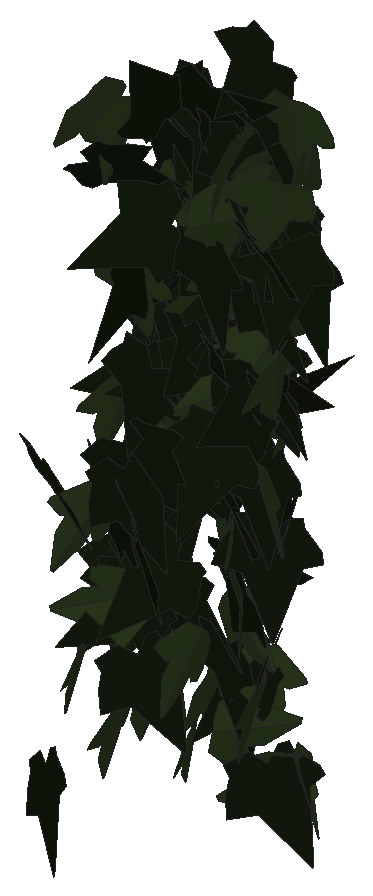
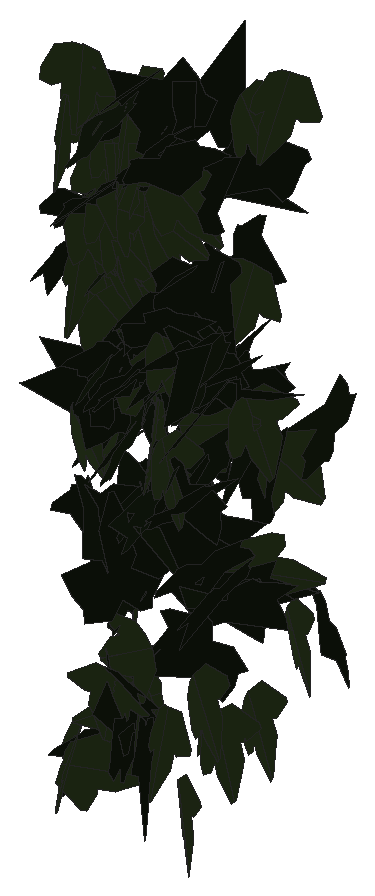
# SketchUp Ruby script. Lengths in inches.
U = 1.inch
M = Sketchup.active_model
def pt(a) = Geom::Point3d.new(a.map { |v| v * U })
def face(e, loops, mat)
  f = e.add_face(loops[0].map { |a| pt(a) })
  loops[1..].each { |l| e.add_face(l.map { |a| pt(a) }).erase! }
  f.material = f.back_material = mat if mat
  f
end
# faces: each face lists its corners as indices into pts; further lists are holes
def faces(e, pts, list, mat = nil) = list.each { |f| face(e, (f[0].is_a?(Array) ? f : [f]).map { |l| l.map { |i| pts[i] } }, mat) }
# xy, xz, yz: faces in a plane at the given z, y or x. An outline is a flat list of corners, or four numbers for a rectangle; further outlines are holes
def ring(l) = l.size == 4 ? [[l[0], l[1]], [l[2], l[1]], [l[2], l[3]], [l[0], l[3]]] : l.each_slice(2).to_a
def flat(e, list, mat, &to3) = list.each { |f| face(e, (f[0].is_a?(Array) ? f : [f]).map { |l| ring(l).map { |u, v| to3.(u, v) } }, mat) }
def xy(e, z, list, mat = nil) = flat(e, list, mat) { |x, y| [x, y, z] }
def xz(e, y, list, mat = nil) = flat(e, list, mat) { |x, z| [x, y, z] }
def yz(e, x, list, mat = nil) = flat(e, list, mat) { |y, z| [x, y, z] }
def lines(e, pts, list) = list.each { |a, b| e.add_line(pt(pts[a]), pt(pts[b])) }
# prism: a flat outline (further loops are holes) pulled along v
def prism(e, loops, v, mat = nil)
  f = face(e, loops, mat); d = Geom::Vector3d.new(v.map { |x| x * U })
  f.pushpull(f.normal.samedirection?(d) ? d.length : -d.length)
end
def box(e, o, s, mat = nil) = prism(e, [[o, [o[0] + s[0], o[1], o[2]], [o[0] + s[0], o[1] + s[1], o[2]], [o[0], o[1] + s[1], o[2]]]], [0, 0, s[2]], mat)
def at(x, y, z, deg = 0) = Geom::Transformation.translation(pt([x, y, z])) * Geom::Transformation.rotation(ORIGIN, Z_AXIS, deg.degrees)
def axes(o, x, y, z) = Geom::Transformation.new([*x, 0, *y, 0, *z, 0, *pt(o).to_a, 1])
def part(name) = M.definitions.add(name)
# library, detail: a bought-in or finely detailed component or shape, given as its bounding box
def library(name, o, s) = part(name).tap { |d| box(d.entities, o, s) }
def detail(e, o, s) = box(e.add_group.entities, o, s)
def put(e, d, t, mat = nil) = e.add_instance(d, t).tap { |i| i.material = mat if mat }
def group(e, t, mat = nil) = e.add_group.tap { |g| g.transformation = t; g.material = mat if mat }.entities
root = M.entities
M.materials.add("efeu1").color = [18, 25, 13]
M.materials.add("efeu2").color = [43, 57, 29]
c1 = part("ivyleaf_9")
p = [[1.54,2.16,1.25],[1.36,2.04,1.19],[-0.21,0.99,0.68],[-0.71,1.11,0.82],[-0.85,0.86,0.67],[-0.8,0.17,0.21],
  [-0.9,-0.01,0.1],[-0.67,-0.16,-0.02],[-0.08,-0.08,-0.05],[-0.03,-0.6,-0.4],[0.65,-0.88,-0.66],[0.83,-0.6,-0.49],
  [1.29,-0.42,-0.43],[1.8125,-0.07,-0.26],[1.21,0.44,0.15]]
faces(c1.entities,p,[[0,1,2,3,4,5,6,7,8,9,10,11,12,13,14]],"efeu1")
c2 = part("ivyleaf_10")
p = [[0,0.5,-0.03],[-0.0625,2.02,-0.43],[-0.19,2.01,-0.46],[-0.54,1.05,-0.29],[-0.52,0.625,-0.18],[-0.83,0.76,-0.28],
  [-1.16,0.64,-0.33],[-1.15,0.33,-0.24],[-0.77,-0.39,0.02],[-0.3,-0.51,0.16],[0.04,-0.48,0.23],[-0.02,2.01,-0.4375],
  [-0.06,2.01,-0.43],[0.04,-0.49,0.23],[0.67,-0.49,0.14],[1.38,0.36,-0.2],[1.375,0.51,-0.24],[0.81,0.65,-0.19],
  [0.62,0.59,-0.15],[0.6,1.09,-0.28],[0.5,1.23,-0.31]]
faces(c2.entities,p,[[0,1,2,3,4,5,6,7,8,9,10],[11,12,0,13,14,15,16,17,18,19,20]],"efeu2")
put(root,c1,axes([25.81,219.31,224.23],[-0.18904,-0.04184,-0.46099],[0.46288,-0.01554,-0.1884],[0.00144,-0.498,0.04461]))
put(root,c2,axes([27.44,220.39,226.23],[-0.01379,-0.37116,0.33473],[0.11301,-0.32851,-0.3596],[0.48687,0.06574,0.09295]))
put(root,c1,axes([26.5625,220.48,227.02],[0.04822,-0.11383,0.48448],[0.15449,-0.45927,-0.12329],[0.47308,0.16159,-0.00912]))
put(root,c1,axes([24.8,220.53,228.01],[0.28782,-0.34234,0.22352],[0.138,-0.17596,-0.44721],[0.38486,0.31912,-0.0068]))
put(root,c2,axes([25.41,220.82,227.49],[-0.09514,-0.36129,0.33229],[0.00188,-0.33874,-0.36777],[0.49086,-0.06873,0.06582]))
put(root,c1,axes([26.41,220.55,225.6],[0.03321,-0.38306,-0.31963],[0.02396,0.32119,-0.38244],[0.49832,0.01008,0.03969]))
put(root,c1,axes([26.13,220.63,228.31],[0.07521,-0.41705,-0.26536],[-0.03138,0.26384,-0.42356],[0.49331,0.08037,0.01351]))
put(root,c2,axes([25.125,220.91,225.13],[0.22225,-0.44783,-0.00737],[-0.00287,0.0068,-0.49995],[0.44788,0.22227,0.00045]))
put(root,c1,axes([26,220.79,228.62],[-0.06742,-0.1291,-0.47832],[0.19906,0.43499,-0.14546],[0.45369,-0.21004,-0.00726]))
put(root,c1,axes([25.79,220.86,228.05],[0.39057,-0.12931,-0.28413],[-0.27142,0.08416,-0.4114],[0.15422,0.4756,-0.00445]))
put(root,c2,axes([25.64,221.24,225.96],[0.10725,0.03356,-0.48721],[-0.44387,-0.20131,-0.11158],[-0.20365,0.45645,-0.01339]))
put(root,c1,axes([25.75,221,226.95],[0.16378,-0.2526,0.39921],[-0.16659,0.3645,0.29898],[-0.44207,-0.23094,0.03524]))
put(root,c1,axes([26.95,221.34,231.67],[0.14266,-0.47158,0.08521],[0.0193,-0.08318,-0.49265],[0.47883,0.14385,-0.00553]))
put(root,c1,axes([26.23,221.37,231.82],[-0.43879,-0.09642,0.21947],[-0.2121,-0.05714,-0.44916],[0.1117,-0.48728,0.00925]))
put(root,c1,axes([25.61,221.55,230.87],[-0.0735,0.05071,-0.49196],[0.3068,-0.38542,-0.08556],[-0.3879,-0.31445,0.02554]))
put(root,c2,axes([25.1,221.14,233.39],[-0.1399,-0.41319,-0.24434],[0.09004,0.2274,-0.4361],[0.47151,-0.16602,0.01078]))
put(root,c1,axes([25.71,221.68,229.26],[-0.04681,-0.44308,0.2269],[0.0125,-0.22888,-0.44436],[0.49765,-0.03592,0.0325]))
put(root,c1,axes([26.15,221.61,226.52],[-0.4073,-0.27121,0.10272],[-0.08761,-0.05376,-0.48932],[0.27646,-0.4166,-0.00373]))
put(root,c1,axes([25.68,221.7,225.74],[-0.29758,-0.24734,0.31665],[-0.23457,-0.21297,-0.38681],[0.32622,-0.37877,0.01071]))
put(root,c2,axes([25.38,221.55,233.18],[0.02209,-0.46526,0.18178],[0.06664,-0.17759,-0.46262],[0.49505,0.04466,0.05417]))
put(root,c2,axes([25.36,221.44,223.99],[0.1074,-0.48763,0.02618],[0.00063,-0.02667,-0.49929],[0.48833,0.10728,-0.00511]))
put(root,c1,axes([25.19,221.11,232.55],[0.40335,0.2125,0.2053],[0.17439,0.10923,-0.45569],[-0.23852,0.43922,0.014]))
put(root,c1,axes([26.89,221.72,228.6],[-0.34885,-0.35579,-0.04139],[0.02971,0.02884,-0.49828],[0.35696,-0.35012,0.00102]))
put(root,c1,axes([27.27,222.03,229.15],[-0.09536,-0.26151,0.41535],[-0.15206,-0.38656,-0.2783],[0.46667,-0.17939,-0.00581]))
put(root,c2,axes([26.94,221.83,232.96],[0.22417,-0.41973,0.15355],[0.07269,-0.13526,-0.47584],[0.44098,0.23566,0.00038]))
put(root,c2,axes([25.14,221.79,228.75],[-0.07663,-0.48144,0.1111],[-0.00512,-0.11164,-0.48735],[0.49407,-0.07582,0.01218]))
put(root,c2,axes([26.85,221.33,232.11],[-0.054,-0.09278,-0.48834],[0.24653,0.42155,-0.10735],[0.43163,-0.25237,0.00021]))
put(root,c2,axes([25.32,221.69,230.65],[-0.49774,0.00252,-0.04744],[0.04743,-0.00113,-0.49774],[-0.00261,-0.49999,0.00088]))
put(root,c1,axes([25.43,221.98,225.99],[-0.33292,-0.36474,-0.07828],[0.06171,0.04963,-0.49369],[0.36791,-0.33838,0.01197]))
put(root,c1,axes([25.68,222,233.05],[0.19902,0.17508,0.42395],[-0.30783,-0.29163,0.26494],[0.34005,-0.36647,-0.00829]))
put(root,c1,axes([25.25,222.11,225.99],[-0.31182,-0.37943,0.09381],[-0.05983,-0.07226,-0.49112],[0.38625,-0.3175,-0.00034]))
put(root,c2,axes([27.73,221.89,232.59],[-0.36147,-0.31379,0.14448],[-0.10382,-0.10077,-0.47861],[0.32949,-0.37601,0.00769]))
put(root,c2,axes([26,221.87,228.33],[-0.12966,0.03247,-0.4818],[-0.47823,0.06057,0.13278],[0.06699,0.49525,0.01535]))
put(root,c1,axes([25.49,221.99,228.27],[0.37885,-0.27455,0.17634],[0.14255,-0.1038,-0.46787],[0.29352,0.40478,-0.00037]))
put(root,c2,axes([27.35,222.04,227.98],[-0.29803,0.31399,-0.25018],[0.16913,-0.18439,-0.43289],[-0.36411,-0.34266,0.00369]))
put(root,c1,axes([26.65,222.28,229.24],[0.39155,-0.27756,-0.14019],[0.11367,-0.08207,0.47994],[-0.28943,-0.40771,-0.00117]))
put(root,c2,axes([26.75,222.13,231.03],[-0.07618,-0.48051,0.11535],[0.01731,-0.11923,-0.48527],[0.49386,-0.06994,0.0348]))
put(root,c1,axes([25.64,222.33,229.01],[-0.37326,-0.07606,0.32387],[-0.26354,-0.22947,-0.35762],[0.20304,-0.43767,0.13122]))
put(root,c2,axes([27.54,222.02,229.8],[0.04755,-0.47944,-0.13372],[0.0118,0.13538,-0.48118],[0.49759,0.0426,0.02419]))
put(root,c2,axes([27.16,222.29,232.44],[-0.04919,-0.44271,0.22713],[-0.0041,-0.22787,-0.44504],[0.49756,-0.04565,0.01879]))
put(root,c1,axes([27.33,222.35,231.21],[0.32566,-0.37936,0.00614],[0.00075,0.00873,0.49992],[-0.37941,-0.3256,0.00625]))
put(root,c2,axes([26.59,222.47,228.98],[-0.07324,0.02485,0.49398],[-0.05974,-0.49616,0.01611],[0.49099,-0.05666,0.07564]))
put(root,c1,axes([27.09,222.31,228.08],[0.0495,-0.49754,-0.00262],[-0.00024,0.00261,-0.49999],[0.49754,0.0495,0.00002]))
put(root,c1,axes([26.82,222.32,232.85],[0.0026,-0.49831,-0.04104],[0.00312,0.04106,-0.4983],[0.49998,0.00234,0.00333]))
put(root,c2,axes([27.14,222.39,229.9],[-0.23714,-0.33155,0.28955],[-0.01137,-0.32417,-0.38051],[0.44004,-0.18705,0.14621]))
put(root,c1,axes([26.66,222.45,227.01],[0.03602,-0.26441,0.42284],[0.17524,-0.39019,-0.25892],[0.4669,0.16685,0.06456]))
put(root,c2,axes([26.92,222.03,225.99],[0.29568,-0.3039,-0.26498],[-0.06469,0.28859,-0.40315],[0.39798,0.27269,0.13134]))
put(root,c2,axes([27.03,222.3,224.49],[0.20793,-0.44947,0.06883],[0.02559,-0.064,-0.49523],[0.45399,0.20947,-0.00361]))
put(root,c1,axes([26.33,222.42,232.73],[0.22631,-0.41067,0.17359],[0.06957,-0.15976,-0.46865],[0.44039,0.23628,-0.01517]))
put(root,c2,axes([26.78,221.98,226.6],[0.06002,-0.00582,0.49635],[-0.4246,0.25838,0.05437],[-0.25712,-0.42803,0.02607]))
put(root,c1,axes([25.75,222.29,230.9375],[-0.04195,0.3771,-0.32563],[0.04589,-0.32247,-0.37935],[-0.49612,-0.06171,-0.00756]))
put(root,c1,axes([27.25,222.37,227],[-0.25743,-0.36093,-0.23121],[0.12767,0.1929,-0.44327],[0.40918,-0.28726,-0.00716]))
put(root,c1,axes([26.99,222.26,230.75],[0.28959,-0.3911,-0.1148],[-0.0162,0.12968,-0.48262],[0.40728,0.28325,0.06244]))
put(root,c1,axes([27.48,222.42,231.47],[-0.31228,-0.34456,-0.18374],[0.12454,0.1351,-0.46501],[0.37009,-0.3362,0.00145]))
put(root,c2,axes([26.86,222.4375,231.29],[-0.02277,-0.46727,0.17647],[0.04644,-0.17787,-0.46498],[0.49732,-0.00479,0.0515]))
put(root,c1,axes([25.9375,222.67,229.31],[-0.13966,-0.3149,0.36239],[-0.01691,-0.37396,-0.33147],[0.4798,-0.10484,0.09381]))
put(root,c2,axes([25.44,222.43,224.54],[-0.21114,0.2378,-0.38584],[0.23092,-0.30982,-0.31731],[-0.39,-0.31219,0.021]))
put(root,c1,axes([26.34,222.54,224.86],[0.11025,-0.45653,0.17155],[0.06544,-0.16044,-0.46902],[0.48328,0.12587,0.02437]))
put(root,c2,axes([25.23,222.35,224.11],[0.00027,-0.49932,0.02614],[0.00009,-0.02614,-0.49932],[0.5,0.00027,0.00008]))
put(root,c1,axes([26.18,222.65,228.58],[-0.10334,-0.4344,0.22499],[0.07044,-0.24077,-0.43251],[0.48411,-0.0577,0.11096]))
put(root,c1,axes([26.55,222.66,225.6875],[-0.04306,-0.24404,0.43427],[0.09256,-0.43222,-0.23371],[0.48947,0.06027,0.0824]))
put(root,c1,axes([26.3,222.31,228.28],[-0.07526,0.3876,0.30676],[0.0076,-0.30935,0.39274],[0.49424,0.06378,0.04068]))
put(root,c1,axes([25.95,222.3,233.09],[0.12133,-0.06883,0.48015],[0.45644,-0.15129,-0.13703],[0.16415,0.47156,0.02612]))
put(root,c2,axes([26.27,222.2,231.45],[0.04551,-0.02293,-0.4974],[-0.42376,0.26047,-0.05078],[0.26145,0.42618,0.00427]))
put(root,c2,axes([26.01,222.42,232.15],[-0.2847,-0.07184,0.4047],[-0.38217,-0.13494,-0.2928],[0.1513,-0.47606,0.02192]))
put(root,c2,axes([27,222.42,232.59],[-0.04731,-0.49776,0.00073],[-0.00019,-0.00071,-0.5],[0.49776,-0.04731,-0.00012]))
put(root,c1,axes([25.86,222.33,231.98],[0.1111,-0.09005,0.47911],[-0.36304,0.31268,0.14295],[-0.32536,-0.37964,0.00409]))
put(root,c1,axes([26.67,222.63,228.19],[0.11847,-0.47794,0.08681],[0.00375,-0.08845,-0.4921],[0.48575,0.11725,-0.01738]))
put(root,c1,axes([25.21,222.77,229.5],[-0.1841,-0.42041,0.19841],[-0.02048,-0.20586,-0.4552],[0.46442,-0.17572,0.05858]))
put(root,c1,axes([27.15,222.42,223.37],[0.0051,-0.4083,-0.28856],[0.07924,0.28559,-0.40269],[0.49366,-0.04163,0.06762]))
put(root,c2,axes([26.72,222.11,223.97],[-0.04493,-0.06391,-0.49386],[0.3304,0.36718,-0.07757],[0.37258,-0.33331,0.00924]))
put(root,c2,axes([26.99,222.51,231.65],[-0.09029,-0.4888,0.05402],[-0.00199,-0.05456,-0.49701],[0.49178,-0.08996,0.0079]))
put(root,c1,axes([26.18,222.79,232.7],[-0.14055,-0.44229,0.18608],[-0.01261,-0.19042,-0.46215],[0.47967,-0.1346,0.04238]))
put(root,c1,axes([25.4,222.38,225.42],[-0.01048,-0.09929,-0.48993],[0.35565,0.34288,-0.0771],[0.35129,-0.35011,0.06344]))
put(root,c1,axes([26.44,222.81,229.18],[-0.13441,-0.46236,0.13473],[0.0244,-0.14624,-0.47751],[0.48098,-0.12179,0.06188]))
put(root,c2,axes([27.56,222.46,233.53],[-0.49875,0.01025,0.03377],[-0.03463,-0.0497,-0.49632],[-0.00681,-0.49742,0.05029]))
put(root,c2,axes([26.43,222.86,231.84],[0.04557,-0.25474,0.42782],[0.2628,-0.35259,-0.23794],[0.42292,0.24655,0.10175]))
put(root,c2,axes([27.27,222.77,223.07],[0.09467,0.09864,-0.48094],[-0.41707,-0.24225,-0.13179],[-0.25901,0.42613,0.03642]))
put(root,c2,axes([26.89,222.57,230.87],[0.43465,-0.13533,-0.2068],[-0.19331,0.07451,-0.45506],[0.15399,0.47553,0.01245]))
put(root,c2,axes([26.72,222.43,232.91],[0.13899,-0.41049,-0.24936],[0.01582,0.26336,-0.42472],[0.48003,0.11017,0.0862]))
put(root,c1,axes([26.86,222.7,229.4],[0.27461,-0.41608,0.03834],[0.02263,-0.031,-0.49852],[0.41723,0.27553,0.0018]))
put(root,c2,axes([27.12,222.76,231.48],[-0.11057,-0.44214,0.20563],[-0.04076,-0.20173,-0.45568],[0.48591,-0.11754,0.00856]))
put(root,c1,axes([26.53,222.84,223.42],[-0.02189,0.14815,0.47705],[-0.11112,-0.46698,0.13992],[0.487,-0.09989,0.05337]))
put(root,c1,axes([25.65,222.74,226.75],[0.41357,-0.02444,0.27993],[-0.27981,0.00989,0.41426],[-0.02579,-0.4993,-0.00549]))
put(root,c1,axes([26.98,222.85,231.85],[-0.1777,-0.46725,-0.01009],[0.00402,0.00926,-0.4999],[0.46734,-0.17775,0.00047]))
put(root,c1,axes([26.76,222.61,229.47],[-0.02629,-0.39355,-0.30728],[0.1034,0.29675,-0.38891],[0.48848,-0.084,0.06578]))
put(root,c1,axes([25.6,222.59,227.83],[-0.15933,-0.12196,-0.45797],[0.36694,0.27404,-0.20064],[0.29995,-0.40003,0.00218]))
put(root,c1,axes([26.45,222.83,229.31],[-0.03199,-0.49796,-0.03175],[0.00101,0.03175,-0.49899],[0.49897,-0.03199,-0.00103]))
put(root,c2,axes([26.85,222.62,232.33],[-0.44809,-0.2077,0.07794],[-0.06717,-0.04038,-0.49382],[0.21143,-0.45302,0.00828]))
put(root,c1,axes([27.1,223.04,231.76],[-0.23273,-0.32327,0.30222],[-0.01462,-0.33566,-0.3703],[0.44229,-0.1812,0.14678]))
put(root,c1,axes([25.48,222.98,227.72],[-0.16961,-0.45211,0.12973],[0.02309,-0.14574,-0.47773],[0.46979,-0.15606,0.07032]))
put(root,c1,axes([25.71,222.35,226.46],[-0.21576,0.44845,-0.04832],[-0.02988,0.03924,0.49756],[0.45006,0.2176,0.00987]))
put(root,c2,axes([25.83,222.72,228.24],[0.0485,-0.49758,0.00787],[0.00281,-0.00763,-0.49993],[0.49763,0.04854,0.00206]))
put(root,c1,axes([26.68,222.8125,224.58],[-0.49812,0.01618,-0.04023],[0.04016,-0.00255,-0.49838],[-0.01634,-0.49973,0.00124]))
put(root,c1,axes([27.38,222.8,231.04],[0.12139,-0.47292,-0.10776],[-0.03416,0.10247,-0.48819],[0.48384,0.12588,-0.00744]))
put(root,c1,axes([25.14,222.86,226.89],[-0.03297,-0.48783,-0.10457],[0.02368,0.10315,-0.48867],[0.49835,-0.03717,0.0163]))
put(root,c1,axes([26.38,222.51,223.76],[0.19087,-0.01002,-0.46203],[-0.45604,0.07685,-0.19006],[0.07482,0.49396,0.0202]))
put(root,c2,axes([27.46,222.52,230.55],[0.02067,-0.39703,-0.30321],[-0.0124,0.30297,-0.39756],[0.49942,0.02396,0.00268]))
put(root,c1,axes([25.07,222.9,229.76],[0.26286,-0.37548,0.1998],[0.12346,-0.1574,-0.45824],[0.40702,0.29023,0.00996]))
put(root,c1,axes([26.3,223.0625,228.34],[0.08581,-0.36082,0.33533],[0.07036,-0.32791,-0.37084],[0.48753,0.11083,-0.0055]))
put(root,c1,axes([26.73,222.84,228.93],[0.15991,-0.13593,0.45382],[0.36744,-0.26674,-0.20937],[0.29902,0.40047,0.01458]))
put(root,c1,axes([25.93,222.79,230.72],[0.11308,-0.45214,-0.18107],[-0.02738,0.17969,-0.46579],[0.48627,0.11526,0.01588]))
put(root,c1,axes([25.71,222.99,232.94],[-0.27656,-0.41527,-0.03266],[0.01679,0.02806,-0.49893],[0.41621,-0.27706,-0.00158]))
put(root,c2,axes([25.73,222.87,230.02],[-0.02977,-0.49067,0.09141],[-0.00959,-0.09099,-0.49156],[0.49902,-0.03102,-0.004]))
put(root,c1,axes([26.6875,223.02,233.02],[0.10217,-0.44965,0.19334],[0.13243,-0.16474,-0.45312],[0.47119,0.1438,0.08543]))
put(root,c2,axes([26.11,222.59,228.68],[0.20388,-0.35782,-0.28354],[-0.00612,0.30836,-0.39354],[0.45651,0.16394,0.12136]))
put(root,c1,axes([26.46,222.91,226],[0.4964,0.02013,0.05641],[-0.05641,-0.0012,0.49681],[0.02014,-0.49959,0.00108]))
put(root,c2,axes([26.2,222.89,225.25],[-0.25993,0.08082,-0.41941],[0.36184,-0.21921,-0.2665],[-0.22696,-0.44206,0.05547]))
put(root,c2,axes([27.48,222.7,223.29],[-0.29948,0.39664,0.05466],[-0.03692,0.04061,-0.49698],[-0.39868,-0.30171,0.00496]))
put(root,c1,axes([25.29,222.41,229.89],[0.11702,0.39662,0.28107],[0.08192,0.26888,-0.41351],[-0.47916,0.14283,-0.00206]))
put(root,c1,axes([25.85,223.09,230.41],[-0.40629,-0.28086,0.07774],[-0.0573,-0.05377,-0.49379],[0.28573,-0.41015,0.01151]))
put(root,c1,axes([25.42,222.76,230.06],[0.1674,-0.37575,-0.28424],[0.02028,0.30711,-0.39404],[0.47071,0.1204,0.11806]))
put(root,c2,axes([25.09,222.94,225],[0.12324,-0.48093,0.05928],[0.01578,-0.05716,-0.49647],[0.48432,0.12424,0.00109]))
put(root,c1,axes([24.82,222.88,226.65],[0.18603,-0.43824,-0.15276],[-0.03971,0.14894,-0.47565],[0.4624,0.1891,0.02061]))
put(root,c1,axes([26.99,222.47,228.76],[-0.00224,0.40837,-0.2885],[-0.03924,0.28747,0.40721],[0.49845,0.02447,0.03076]))
put(root,c1,axes([26.48,223.26,233.57],[-0.21792,-0.32781,0.3083],[-0.00656,-0.3402,-0.36636],[0.44997,-0.16372,0.14397]))
put(root,c1,axes([25.09,223.04,229.23],[0.16082,-0.47145,0.04325],[0.01202,-0.04159,-0.49812],[0.47328,0.16125,-0.00204]))
put(root,c1,axes([25.86,223,227.62],[0.28851,-0.39295,0.11115],[0.06834,-0.08772,-0.48748],[0.40261,0.29648,0.00309]))
put(root,c2,axes([26.61,222.85,224.55],[0.45706,0.1552,0.13041],[0.12037,0.05105,-0.4826],[-0.16311,0.47255,0.00931]))
put(root,c2,axes([27.57,222.71,232.85],[0.12541,-0.40859,-0.25947],[0.00509,0.26913,-0.42136],[0.48399,0.10304,0.07167]))
put(root,c2,axes([25.48,222.83,223.2],[0.21078,-0.433,-0.13449],[-0.02414,0.13738,-0.48015],[0.45276,0.2089,0.03701]))
put(root,c2,axes([27.05,223.05,228.52],[0.18595,-0.43046,0.17356],[0.06567,-0.16069,-0.4689],[0.45947,0.19718,-0.00323]))
put(root,c1,axes([26.75,222.49,224.06],[0.04114,0.10504,0.48711],[0.03987,0.4865,-0.10828],[-0.49671,0.04775,0.03165]))
put(root,c2,axes([25.86,222.7,224.12],[0.04454,-0.40742,-0.28639],[0.01743,0.28864,-0.4079],[0.49771,0.02636,0.03992]))
put(root,c1,axes([27.1875,222.51,226.69],[-0.011,0.21112,0.45311],[-0.04403,0.45105,-0.21123],[-0.49794,-0.04455,0.00866]))
